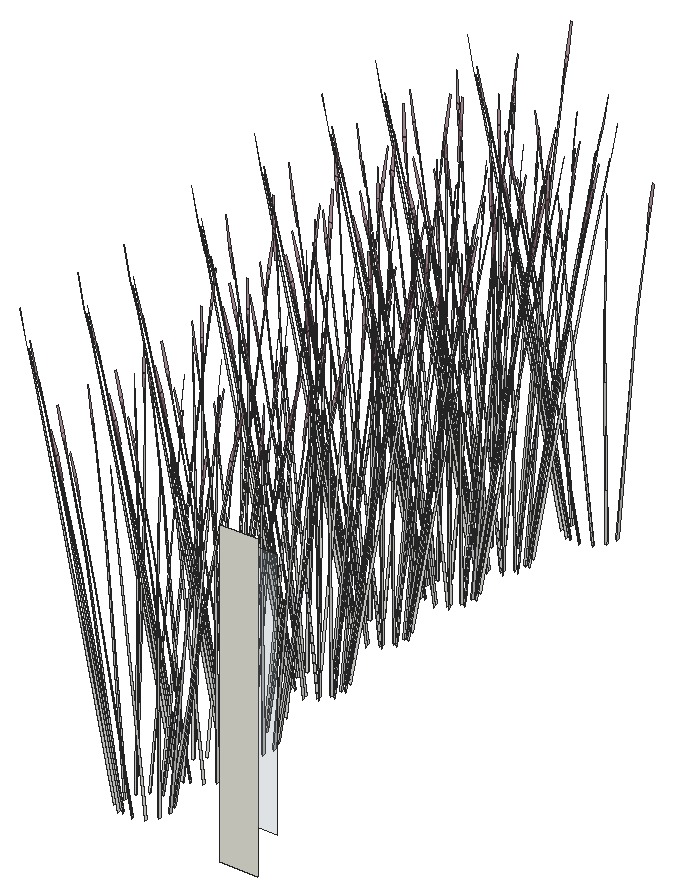
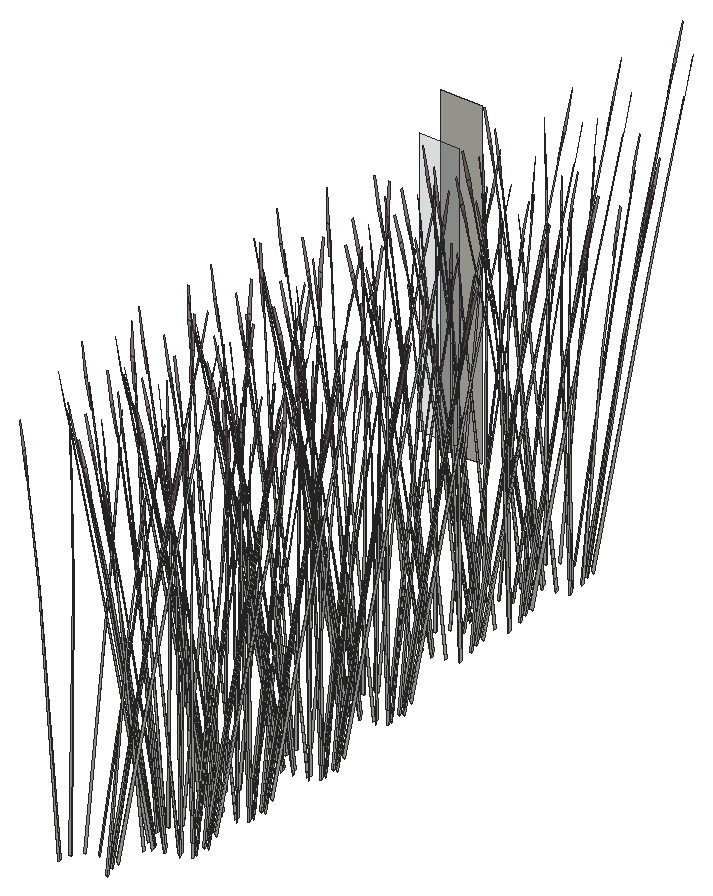
# SketchUp Ruby script. Lengths in inches.
U = 1.inch
M = Sketchup.active_model
def pt(a) = Geom::Point3d.new(a.map { |v| v * U })
def face(e, loops, mat)
  f = e.add_face(loops[0].map { |a| pt(a) })
  loops[1..].each { |l| e.add_face(l.map { |a| pt(a) }).erase! }
  f.material = f.back_material = mat if mat
  f
end
# faces: each face lists its corners as indices into pts; further lists are holes
def faces(e, pts, list, mat = nil) = list.each { |f| face(e, (f[0].is_a?(Array) ? f : [f]).map { |l| l.map { |i| pts[i] } }, mat) }
# xy, xz, yz: faces in a plane at the given z, y or x. An outline is a flat list of corners, or four numbers for a rectangle; further outlines are holes
def ring(l) = l.size == 4 ? [[l[0], l[1]], [l[2], l[1]], [l[2], l[3]], [l[0], l[3]]] : l.each_slice(2).to_a
def flat(e, list, mat, &to3) = list.each { |f| face(e, (f[0].is_a?(Array) ? f : [f]).map { |l| ring(l).map { |u, v| to3.(u, v) } }, mat) }
def xy(e, z, list, mat = nil) = flat(e, list, mat) { |x, y| [x, y, z] }
def xz(e, y, list, mat = nil) = flat(e, list, mat) { |x, z| [x, y, z] }
def yz(e, x, list, mat = nil) = flat(e, list, mat) { |y, z| [x, y, z] }
def lines(e, pts, list) = list.each { |a, b| e.add_line(pt(pts[a]), pt(pts[b])) }
# prism: a flat outline (further loops are holes) pulled along v
def prism(e, loops, v, mat = nil)
  f = face(e, loops, mat); d = Geom::Vector3d.new(v.map { |x| x * U })
  f.pushpull(f.normal.samedirection?(d) ? d.length : -d.length)
end
def box(e, o, s, mat = nil) = prism(e, [[o, [o[0] + s[0], o[1], o[2]], [o[0] + s[0], o[1] + s[1], o[2]], [o[0], o[1] + s[1], o[2]]]], [0, 0, s[2]], mat)
def at(x, y, z, deg = 0) = Geom::Transformation.translation(pt([x, y, z])) * Geom::Transformation.rotation(ORIGIN, Z_AXIS, deg.degrees)
def axes(o, x, y, z) = Geom::Transformation.new([*x, 0, *y, 0, *z, 0, *pt(o).to_a, 1])
def part(name) = M.definitions.add(name)
# library, detail: a bought-in or finely detailed component or shape, given as its bounding box
def library(name, o, s) = part(name).tap { |d| box(d.entities, o, s) }
def detail(e, o, s) = box(e.add_group.entities, o, s)
def put(e, d, t, mat = nil) = e.add_instance(d, t).tap { |i| i.material = mat if mat }
def group(e, t, mat = nil) = e.add_group.tap { |g| g.transformation = t; g.material = mat if mat }.entities
root = M.entities
M.materials.add("D01_Frost_White").color = [238, 238, 227]
M.materials.add("Glass_Basic_01").color = [161, 173, 186]
M.materials["Glass_Basic_01"].alpha = 0.25
M.materials.add("LightPink_Translucent").color = [144, 107, 117]
M.materials["LightPink_Translucent"].alpha = 0.75
c1 = part("blade")
p = [[2.15,0.21,22],[0,0.17,0],[0.09,0.45,0],[2.18,0.31,22],[2.29,0.31,22],[0.38,0.45,0],
  [2.48,0.24,33],[2.49,0.24,33],[2.48,0.22,33]]
faces(c1.entities,p,[[0,1,2,3],[4,5,2,3],[6,3,4,7],[8,0,3,6]])
c2 = part("seeds")
p = [[0.3,-0.1,1.38],[-0.01,-0.03,1.59],[-0.01,-0.03,0.03],[0.14,-0.07,-0.07],[0.29,-0.03,3],[0.15,0.01,3.11]]
faces(c2.entities,p,[[0,1,2,3],[1,0,4,5]],"LightPink_Translucent")
c3 = part("blade with seeds")
put(c3.entities,c1,at(0,0,0))
put(c3.entities,c2,axes([2.4,0.25,30.99],[1.5799,-0.05474,1.17369],[-0.12525,1.92788,0.29478],[-0.07173,-0.02425,1.56792]))
xz(root,373,[[439,156,442,180]],"D01_Frost_White")
xz(root,375,[[439,158,442,178]],"Glass_Basic_01")
put(root,c3,axes([428.4,376.04,154.3],[0.45651,-0.12123,0.45419],[0.07923,0.47555,0.3745],[-0.10736,-0.14016,0.93983]))
put(root,c3,axes([429.43,376.43,154.27],[-0.12355,0.36271,0.29918],[-0.36044,-0.10579,-0.38624],[-0.03305,-0.14603,0.73904]))
put(root,c3,axes([430.21,376.84,154.27],[-0.27728,0.24833,0.29918],[-0.26248,-0.28355,-0.38624],[0.03994,-0.14407,0.73904]))
put(root,c3,axes([428.56,376.49,154.27],[0.06329,0.37991,0.29918],[-0.36182,0.10032,-0.38624],[-0.09718,-0.10887,0.73904]))
put(root,c3,axes([427.48,376.74,154.3],[0.33843,-0.34808,0.45419],[0.29188,0.36965,0.3745],[-0.15878,-0.06421,0.93983]))
put(root,c3,axes([430.6875,377.61,154.27],[-0.35672,0.06741,0.29918],[-0.09419,-0.38534,-0.38624],[0.10222,-0.1035,0.73904]))
put(root,c3,axes([427.84,377,154.27],[0.23317,0.29531,0.29918],[-0.26625,0.27955,-0.38624],[-0.13527,-0.04253,0.73904]))
put(root,c3,axes([430.75,378.53,154.27],[-0.34057,-0.13158,0.29918],[0.09933,-0.38387,-0.38624],[0.13712,-0.0352,0.73904]))
put(root,c3,axes([427.46,377.83,154.27],[0.34057,0.13158,0.29918],[-0.09933,0.38387,-0.38624],[-0.13712,0.0352,0.73904]))
put(root,c3,axes([428.4,381.79,154.3],[0.45651,-0.12123,0.45419],[0.07923,0.47555,0.3745],[-0.10736,-0.14016,0.93983]))
put(root,c3,axes([430.36,379.36,154.27],[-0.23317,-0.29531,0.29918],[0.26625,-0.27955,-0.38624],[0.13527,0.04253,0.73904]))
put(root,c3,axes([429.43,382.18,154.27],[-0.12355,0.36271,0.29918],[-0.36044,-0.10579,-0.38624],[-0.03305,-0.14603,0.73904]))
put(root,c3,axes([430.21,382.59,154.27],[-0.27728,0.24833,0.29918],[-0.26248,-0.28355,-0.38624],[0.03994,-0.14407,0.73904]))
put(root,c3,axes([427.52,378.75,154.27],[0.35672,-0.06741,0.29918],[0.09419,0.38534,-0.38624],[-0.10222,0.1035,0.73904]))
put(root,c3,axes([428.56,382.24,154.27],[0.06329,0.37991,0.29918],[-0.36182,0.10032,-0.38624],[-0.09718,-0.10887,0.73904]))
put(root,c3,axes([427.48,382.49,154.3],[0.33843,-0.34808,0.45419],[0.29188,0.36965,0.3745],[-0.15878,-0.06421,0.93983]))
put(root,c3,axes([426.71,379.85,154.77],[0.36162,0.1259,-0.05481],[-0.11124,0.3875,-0.2485],[-0.05915,0.05883,0.81966]))
put(root,c3,axes([429.64,379.87,154.27],[-0.06329,-0.37991,0.29918],[0.36182,-0.10032,-0.38624],[0.09718,0.10887,0.73904]))
put(root,c3,axes([430.6875,383.35,154.27],[-0.35672,0.06741,0.29918],[-0.09419,-0.38534,-0.38624],[0.10222,-0.1035,0.73904]))
put(root,c3,axes([428,379.52,154.27],[0.27728,-0.24833,0.29918],[0.26248,0.28355,-0.38624],[-0.03994,0.14407,0.73904]))
put(root,c3,axes([428.78,379.93,154.27],[0.12355,-0.36271,0.29918],[0.36044,0.10579,-0.38624],[0.03305,0.14603,0.73904]))
put(root,c3,axes([429.26,381.22,154.77],[0.28319,-0.27058,-0.05481],[0.25948,0.29635,-0.2485],[0.01827,0.08397,0.81966]))
put(root,c3,axes([427.84,382.75,154.27],[0.23317,0.29531,0.29918],[-0.26625,0.27955,-0.38624],[-0.13527,-0.04253,0.73904]))
put(root,c3,axes([428.77,380.23,154.28],[-0.4038,-0.12331,0.45013],[0.13808,-0.40538,0.37115],[0.02427,0.15942,0.93144]))
put(root,c3,axes([430.75,384.28,154.27],[-0.34057,-0.13158,0.29918],[0.09933,-0.38387,-0.38624],[0.13712,-0.0352,0.73904]))
put(root,c3,axes([428.4,386.36,154.3],[0.45651,-0.12123,0.45419],[0.07923,0.47555,0.3745],[-0.10736,-0.14016,0.93983]))
put(root,c3,axes([427.46,383.58,154.27],[0.34057,0.13158,0.29918],[-0.09933,0.38387,-0.38624],[-0.13712,0.0352,0.73904]))
put(root,c3,axes([429.43,386.75,154.27],[-0.12355,0.36271,0.29918],[-0.36044,-0.10579,-0.38624],[-0.03305,-0.14603,0.73904]))
put(root,c3,axes([430.21,387.16,154.27],[-0.27728,0.24833,0.29918],[-0.26248,-0.28355,-0.38624],[0.03994,-0.14407,0.73904]))
put(root,c3,axes([430.36,385.1,154.27],[-0.23317,-0.29531,0.29918],[0.26625,-0.27955,-0.38624],[0.13527,0.04253,0.73904]))
put(root,c3,axes([428.56,386.81,154.27],[0.06329,0.37991,0.29918],[-0.36182,0.10032,-0.38624],[-0.09718,-0.10887,0.73904]))
put(root,c3,axes([427.48,387.06,154.3],[0.33843,-0.34808,0.45419],[0.29188,0.36965,0.3745],[-0.15878,-0.06421,0.93983]))
put(root,c3,axes([430.6875,387.93,154.27],[-0.35672,0.06741,0.29918],[-0.09419,-0.38534,-0.38624],[0.10222,-0.1035,0.73904]))
put(root,c3,axes([427.52,384.5,154.27],[0.35672,-0.06741,0.29918],[0.09419,0.38534,-0.38624],[-0.10222,0.1035,0.73904]))
put(root,c3,axes([426.71,385.6,154.77],[0.36162,0.1259,-0.05481],[-0.11124,0.3875,-0.2485],[-0.05915,0.05883,0.81966]))
put(root,c3,axes([429.64,385.62,154.27],[-0.06329,-0.37991,0.29918],[0.36182,-0.10032,-0.38624],[0.09718,0.10887,0.73904]))
put(root,c3,axes([427.84,387.32,154.27],[0.23317,0.29531,0.29918],[-0.26625,0.27955,-0.38624],[-0.13527,-0.04253,0.73904]))
put(root,c3,axes([428,385.27,154.27],[0.27728,-0.24833,0.29918],[0.26248,0.28355,-0.38624],[-0.03994,0.14407,0.73904]))
put(root,c3,axes([428.78,385.68,154.27],[0.12355,-0.36271,0.29918],[0.36044,0.10579,-0.38624],[0.03305,0.14603,0.73904]))
put(root,c3,axes([430.75,388.85,154.27],[-0.34057,-0.13158,0.29918],[0.09933,-0.38387,-0.38624],[0.13712,-0.0352,0.73904]))
put(root,c3,axes([429.26,386.97,154.77],[0.28319,-0.27058,-0.05481],[0.25948,0.29635,-0.2485],[0.01827,0.08397,0.81966]))
put(root,c3,axes([428.77,385.98,154.28],[-0.4038,-0.12331,0.45013],[0.13808,-0.40538,0.37115],[0.02427,0.15942,0.93144]))
put(root,c3,axes([427.46,388.15,154.27],[0.34057,0.13158,0.29918],[-0.09933,0.38387,-0.38624],[-0.13712,0.0352,0.73904]))
put(root,c3,axes([430.36,389.68,154.27],[-0.23317,-0.29531,0.29918],[0.26625,-0.27955,-0.38624],[0.13527,0.04253,0.73904]))
put(root,c3,axes([427.52,389.07,154.27],[0.35672,-0.06741,0.29918],[0.09419,0.38534,-0.38624],[-0.10222,0.1035,0.73904]))
put(root,c3,axes([426.71,390.17,154.77],[0.36162,0.1259,-0.05481],[-0.11124,0.3875,-0.2485],[-0.05915,0.05883,0.81966]))
put(root,c3,axes([429.64,390.1875,154.27],[-0.06329,-0.37991,0.29918],[0.36182,-0.10032,-0.38624],[0.09718,0.10887,0.73904]))
put(root,c3,axes([428,389.84,154.27],[0.27728,-0.24833,0.29918],[0.26248,0.28355,-0.38624],[-0.03994,0.14407,0.73904]))
put(root,c3,axes([427.05,394.79,154.3],[0.45651,-0.12123,0.45419],[0.07923,0.47555,0.3745],[-0.10736,-0.14016,0.93983]))
put(root,c3,axes([428.08,394.875,154],[0.4038,0.12331,0.40553],[-0.13808,0.40538,0.33437],[-0.02427,-0.15942,0.83914]))
put(root,c3,axes([428.78,390.25,154.27],[0.12355,-0.36271,0.29918],[0.36044,0.10579,-0.38624],[0.03305,0.14603,0.73904]))
put(root,c3,axes([429.26,391.54,154.77],[0.28319,-0.27058,-0.05481],[0.25948,0.29635,-0.2485],[0.01827,0.08397,0.81966]))
put(root,c3,axes([428.07,395.17,154.27],[-0.12355,0.36271,0.29918],[-0.36044,-0.10579,-0.38624],[-0.03305,-0.14603,0.73904]))
put(root,c3,axes([429,395.33,154],[0.29182,0.32181,0.40553],[-0.3099,0.27755,0.33437],[0.05383,-0.15098,0.83914]))
put(root,c3,axes([428.77,390.55,154.28],[-0.4038,-0.12331,0.45013],[0.13808,-0.40538,0.37115],[0.02427,0.15942,0.93144]))
put(root,c3,axes([428.85,395.58,154.27],[-0.27728,0.24833,0.29918],[-0.26248,-0.28355,-0.38624],[0.03994,-0.14407,0.73904]))
put(root,c3,axes([427.21,395.24,154.27],[0.06329,0.37991,0.29918],[-0.36182,0.10032,-0.38624],[-0.09718,-0.10887,0.73904]))
put(root,c3,axes([426.12,395.48,154.3],[0.33843,-0.34808,0.45419],[0.29188,0.36965,0.3745],[-0.15878,-0.06421,0.93983]))
put(root,c3,axes([429.33,396.35,154.27],[-0.35672,0.06741,0.29918],[-0.09419,-0.38534,-0.38624],[0.10222,-0.1035,0.73904]))
put(root,c3,axes([429.58,396.21,154],[0.10163,0.43409,0.40553],[-0.39868,0.07534,0.33437],[0.1175,-0.10209,0.83914]))
put(root,c3,axes([426.49,395.75,154.27],[0.23317,0.29531,0.29918],[-0.26625,0.27955,-0.38624],[-0.13527,-0.04253,0.73904]))
put(root,c3,axes([429.39,397.27,154.27],[-0.34057,-0.13158,0.29918],[0.09933,-0.38387,-0.38624],[0.13712,-0.0352,0.73904]))
put(root,c3,axes([425.82,396.57,154],[0.11578,-0.43006,0.40553],[0.38064,0.14706,0.33437],[-0.14969,0.02584,0.83914]))
put(root,c3,axes([429.67,397.28,154],[-0.11578,0.43006,0.40553],[-0.38064,-0.14706,0.33437],[0.14969,-0.02584,0.83914]))
put(root,c3,axes([426.1,396.58,154.27],[0.34057,0.13158,0.29918],[-0.09933,0.38387,-0.38624],[-0.13712,0.0352,0.73904]))
put(root,c3,axes([429.01,398.1,154.27],[-0.23317,-0.29531,0.29918],[0.26625,-0.27955,-0.38624],[0.13527,0.04253,0.73904]))
put(root,c3,axes([425.92,397.64,154],[-0.10163,-0.43409,0.40553],[0.39868,-0.07534,0.33437],[-0.1175,0.10209,0.83914]))
put(root,c3,axes([426.16,397.5,154.27],[0.35672,-0.06741,0.29918],[0.09419,0.38534,-0.38624],[-0.10222,0.1035,0.73904]))
put(root,c3,axes([429.25,398.25,154],[-0.30217,0.31079,0.40553],[-0.2606,-0.33005,0.33437],[0.14177,0.05733,0.83914]))
put(root,c3,axes([425.96,402.37,154.3],[0.45651,-0.12123,0.45419],[0.07923,0.47555,0.3745],[-0.10736,-0.14016,0.93983]))
put(root,c3,axes([426.99,402.46,154],[0.4038,0.12331,0.40553],[-0.13808,0.40538,0.33437],[-0.02427,-0.15942,0.83914]))
put(root,c3,axes([425.35,398.59,154.77],[0.36162,0.1259,-0.05481],[-0.11124,0.3875,-0.2485],[-0.05915,0.05883,0.81966]))
put(root,c3,axes([428.28,398.61,154.27],[-0.06329,-0.37991,0.29918],[0.36182,-0.10032,-0.38624],[0.09718,0.10887,0.73904]))
put(root,c3,axes([426.64,398.27,154.27],[0.27728,-0.24833,0.29918],[0.26248,0.28355,-0.38624],[-0.03994,0.14407,0.73904]))
put(root,c3,axes([426.99,402.75,154.27],[-0.12355,0.36271,0.29918],[-0.36044,-0.10579,-0.38624],[-0.03305,-0.14603,0.73904]))
put(root,c3,axes([427.91,402.91,154],[0.29182,0.32181,0.40553],[-0.3099,0.27755,0.33437],[0.05383,-0.15098,0.83914]))
put(root,c3,axes([426.5,398.52,154],[-0.29182,-0.32181,0.40553],[0.3099,-0.27755,0.33437],[-0.05383,0.15098,0.83914]))
put(root,c3,axes([427.42,398.67,154.27],[0.12355,-0.36271,0.29918],[0.36044,0.10579,-0.38624],[0.03305,0.14603,0.73904]))
put(root,c3,axes([427.77,403.16,154.27],[-0.27728,0.24833,0.29918],[-0.26248,-0.28355,-0.38624],[0.03994,-0.14407,0.73904]))
put(root,c3,axes([427.9,399.97,154.77],[0.28319,-0.27058,-0.05481],[0.25948,0.29635,-0.2485],[0.01827,0.08397,0.81966]))
put(root,c3,axes([428.42,398.875,154],[-0.4076,0.10824,0.40553],[-0.07074,-0.4246,0.33437],[0.09586,0.12514,0.83914]))
put(root,c3,axes([426.125,402.8125,154.27],[0.06329,0.37991,0.29918],[-0.36182,0.10032,-0.38624],[-0.09718,-0.10887,0.73904]))
put(root,c3,axes([425.04,403.0625,154.3],[0.33843,-0.34808,0.45419],[0.29188,0.36965,0.3745],[-0.15878,-0.06421,0.93983]))
put(root,c3,axes([427.41,398.97,154.28],[-0.4038,-0.12331,0.45013],[0.13808,-0.40538,0.37115],[0.02427,0.15942,0.93144]))
put(root,c3,axes([428.25,403.93,154.27],[-0.35672,0.06741,0.29918],[-0.09419,-0.38534,-0.38624],[0.10222,-0.1035,0.73904]))
put(root,c3,axes([428.49,403.78,154],[0.10163,0.43409,0.40553],[-0.39868,0.07534,0.33437],[0.1175,-0.10209,0.83914]))
put(root,c3,axes([425.4,403.33,154.27],[0.23317,0.29531,0.29918],[-0.26625,0.27955,-0.38624],[-0.13527,-0.04253,0.73904]))
put(root,c3,axes([428.3,404.85,154.27],[-0.34057,-0.13158,0.29918],[0.09933,-0.38387,-0.38624],[0.13712,-0.0352,0.73904]))
put(root,c3,axes([424.74,404.15,154],[0.11578,-0.43006,0.40553],[0.38064,0.14706,0.33437],[-0.14969,0.02584,0.83914]))
put(root,c3,axes([428.58,404.86,154],[-0.11578,0.43006,0.40553],[-0.38064,-0.14706,0.33437],[0.14969,-0.02584,0.83914]))
put(root,c3,axes([425.02,404.15,154.27],[0.34057,0.13158,0.29918],[-0.09933,0.38387,-0.38624],[-0.13712,0.0352,0.73904]))
put(root,c3,axes([427.92,405.68,154.27],[-0.23317,-0.29531,0.29918],[0.26625,-0.27955,-0.38624],[0.13527,0.04253,0.73904]))
put(root,c3,axes([426.11,408.92,154.3],[0.45651,-0.12123,0.45419],[0.07923,0.47555,0.3745],[-0.10736,-0.14016,0.93983]))
put(root,c3,axes([427.14,409,154],[0.4038,0.12331,0.40553],[-0.13808,0.40538,0.33437],[-0.02427,-0.15942,0.83914]))
put(root,c3,axes([424.83,405.22,154],[-0.10163,-0.43409,0.40553],[0.39868,-0.07534,0.33437],[-0.1175,0.10209,0.83914]))
put(root,c3,axes([425.08,405.08,154.27],[0.35672,-0.06741,0.29918],[0.09419,0.38534,-0.38624],[-0.10222,0.1035,0.73904]))
put(root,c3,axes([427.13,409.3,154.27],[-0.12355,0.36271,0.29918],[-0.36044,-0.10579,-0.38624],[-0.03305,-0.14603,0.73904]))
put(root,c3,axes([428.05,409.45,154],[0.29182,0.32181,0.40553],[-0.3099,0.27755,0.33437],[0.05383,-0.15098,0.83914]))
put(root,c3,axes([428.16,405.83,154],[-0.30217,0.31079,0.40553],[-0.2606,-0.33005,0.33437],[0.14177,0.05733,0.83914]))
put(root,c3,axes([427.91,409.71,154.27],[-0.27728,0.24833,0.29918],[-0.26248,-0.28355,-0.38624],[0.03994,-0.14407,0.73904]))
put(root,c3,axes([424.27,406.17,154.77],[0.36162,0.1259,-0.05481],[-0.11124,0.3875,-0.2485],[-0.05915,0.05883,0.81966]))
put(root,c3,axes([427.2,406.19,154.27],[-0.06329,-0.37991,0.29918],[0.36182,-0.10032,-0.38624],[0.09718,0.10887,0.73904]))
put(root,c3,axes([426.27,409.36,154.27],[0.06329,0.37991,0.29918],[-0.36182,0.10032,-0.38624],[-0.09718,-0.10887,0.73904]))
put(root,c3,axes([425.18,409.61,154.3],[0.33843,-0.34808,0.45419],[0.29188,0.36965,0.3745],[-0.15878,-0.06421,0.93983]))
put(root,c3,axes([425.56,405.84,154.27],[0.27728,-0.24833,0.29918],[0.26248,0.28355,-0.38624],[-0.03994,0.14407,0.73904]))
put(root,c3,axes([425.41,406.1,154],[-0.29182,-0.32181,0.40553],[0.3099,-0.27755,0.33437],[-0.05383,0.15098,0.83914]))
put(root,c3,axes([426.34,406.25,154.27],[0.12355,-0.36271,0.29918],[0.36044,0.10579,-0.38624],[0.03305,0.14603,0.73904]))
put(root,c3,axes([428.39,410.48,154.27],[-0.35672,0.06741,0.29918],[-0.09419,-0.38534,-0.38624],[0.10222,-0.1035,0.73904]))
put(root,c3,axes([426.82,407.55,154.77],[0.28319,-0.27058,-0.05481],[0.25948,0.29635,-0.2485],[0.01827,0.08397,0.81966]))
put(root,c3,axes([427.34,406.45,154],[-0.4076,0.10824,0.40553],[-0.07074,-0.4246,0.33437],[0.09586,0.12514,0.83914]))
put(root,c3,axes([428.64,410.33,154],[0.10163,0.43409,0.40553],[-0.39868,0.07534,0.33437],[0.1175,-0.10209,0.83914]))
put(root,c3,axes([426.33,406.55,154.28],[-0.4038,-0.12331,0.45013],[0.13808,-0.40538,0.37115],[0.02427,0.15942,0.93144]))
put(root,c3,axes([425.55,409.875,154.27],[0.23317,0.29531,0.29918],[-0.26625,0.27955,-0.38624],[-0.13527,-0.04253,0.73904]))
put(root,c3,axes([428.45,411.4,154.27],[-0.34057,-0.13158,0.29918],[0.09933,-0.38387,-0.38624],[0.13712,-0.0352,0.73904]))
put(root,c3,axes([424.88,410.7,154],[0.11578,-0.43006,0.40553],[0.38064,0.14706,0.33437],[-0.14969,0.02584,0.83914]))
put(root,c3,axes([428.73,411.4,154],[-0.11578,0.43006,0.40553],[-0.38064,-0.14706,0.33437],[0.14969,-0.02584,0.83914]))
put(root,c3,axes([425.16,410.7,154.27],[0.34057,0.13158,0.29918],[-0.09933,0.38387,-0.38624],[-0.13712,0.0352,0.73904]))
put(root,c3,axes([426.04,414.3,154.3],[0.45651,-0.12123,0.45419],[0.07923,0.47555,0.3745],[-0.10736,-0.14016,0.93983]))
put(root,c3,axes([427.07,414.39,154],[0.4038,0.12331,0.40553],[-0.13808,0.40538,0.33437],[-0.02427,-0.15942,0.83914]))
put(root,c3,axes([428.07,412.23,154.27],[-0.23317,-0.29531,0.29918],[0.26625,-0.27955,-0.38624],[0.13527,0.04253,0.73904]))
put(root,c3,axes([427.0625,414.68,154.27],[-0.12355,0.36271,0.29918],[-0.36044,-0.10579,-0.38624],[-0.03305,-0.14603,0.73904]))
put(root,c3,axes([427.98,414.84,154],[0.29182,0.32181,0.40553],[-0.3099,0.27755,0.33437],[0.05383,-0.15098,0.83914]))
put(root,c3,axes([427.84,415.09,154.27],[-0.27728,0.24833,0.29918],[-0.26248,-0.28355,-0.38624],[0.03994,-0.14407,0.73904]))
put(root,c3,axes([424.98,411.77,154],[-0.10163,-0.43409,0.40553],[0.39868,-0.07534,0.33437],[-0.1175,0.10209,0.83914]))
put(root,c3,axes([426.2,414.74,154.27],[0.06329,0.37991,0.29918],[-0.36182,0.10032,-0.38624],[-0.09718,-0.10887,0.73904]))
put(root,c3,axes([425.11,414.99,154.3],[0.33843,-0.34808,0.45419],[0.29188,0.36965,0.3745],[-0.15878,-0.06421,0.93983]))
put(root,c3,axes([425.22,411.625,154.27],[0.35672,-0.06741,0.29918],[0.09419,0.38534,-0.38624],[-0.10222,0.1035,0.73904]))
put(root,c3,axes([428.31,412.38,154],[-0.30217,0.31079,0.40553],[-0.2606,-0.33005,0.33437],[0.14177,0.05733,0.83914]))
put(root,c3,axes([428.32,415.86,154.27],[-0.35672,0.06741,0.29918],[-0.09419,-0.38534,-0.38624],[0.10222,-0.1035,0.73904]))
put(root,c3,axes([424.41,412.72,154.77],[0.36162,0.1259,-0.05481],[-0.11124,0.3875,-0.2485],[-0.05915,0.05883,0.81966]))
put(root,c3,axes([427.34,412.74,154.27],[-0.06329,-0.37991,0.29918],[0.36182,-0.10032,-0.38624],[0.09718,0.10887,0.73904]))
put(root,c3,axes([428.57,415.72,154],[0.10163,0.43409,0.40553],[-0.39868,0.07534,0.33437],[0.1175,-0.10209,0.83914]))
put(root,c3,axes([425.7,412.39,154.27],[0.27728,-0.24833,0.29918],[0.26248,0.28355,-0.38624],[-0.03994,0.14407,0.73904]))
put(root,c3,axes([425.56,412.65,154],[-0.29182,-0.32181,0.40553],[0.3099,-0.27755,0.33437],[-0.05383,0.15098,0.83914]))
put(root,c3,axes([426.48,412.8,154.27],[0.12355,-0.36271,0.29918],[0.36044,0.10579,-0.38624],[0.03305,0.14603,0.73904]))
put(root,c3,axes([425.48,415.26,154.27],[0.23317,0.29531,0.29918],[-0.26625,0.27955,-0.38624],[-0.13527,-0.04253,0.73904]))
put(root,c3,axes([426.96,414.09,154.77],[0.28319,-0.27058,-0.05481],[0.25948,0.29635,-0.2485],[0.01827,0.08397,0.81966]))
put(root,c3,axes([427.48,413,154],[-0.4076,0.10824,0.40553],[-0.07074,-0.4246,0.33437],[0.09586,0.12514,0.83914]))
put(root,c3,axes([426.47,413.1,154.28],[-0.4038,-0.12331,0.45013],[0.13808,-0.40538,0.37115],[0.02427,0.15942,0.93144]))
put(root,c3,axes([428.38,416.78,154.27],[-0.34057,-0.13158,0.29918],[0.09933,-0.38387,-0.38624],[0.13712,-0.0352,0.73904]))
put(root,c3,axes([424.8125,416.08,154],[0.11578,-0.43006,0.40553],[0.38064,0.14706,0.33437],[-0.14969,0.02584,0.83914]))
put(root,c3,axes([428.66,416.79,154],[-0.11578,0.43006,0.40553],[-0.38064,-0.14706,0.33437],[0.14969,-0.02584,0.83914]))
put(root,c3,axes([425.09,416.09,154.27],[0.34057,0.13158,0.29918],[-0.09933,0.38387,-0.38624],[-0.13712,0.0352,0.73904]))
put(root,c3,axes([428.4,420.45,154.3],[0.45651,-0.12123,0.45419],[0.07923,0.47555,0.3745],[-0.10736,-0.14016,0.93983]))
put(root,c3,axes([428,417.61,154.27],[-0.23317,-0.29531,0.29918],[0.26625,-0.27955,-0.38624],[0.13527,0.04253,0.73904]))
put(root,c3,axes([424.91,417.15,154],[-0.10163,-0.43409,0.40553],[0.39868,-0.07534,0.33437],[-0.1175,0.10209,0.83914]))
put(root,c3,axes([429.43,420.84,154.27],[-0.12355,0.36271,0.29918],[-0.36044,-0.10579,-0.38624],[-0.03305,-0.14603,0.73904]))
put(root,c3,axes([425.15,417.01,154.27],[0.35672,-0.06741,0.29918],[0.09419,0.38534,-0.38624],[-0.10222,0.1035,0.73904]))
put(root,c3,axes([430.21,421.25,154.27],[-0.27728,0.24833,0.29918],[-0.26248,-0.28355,-0.38624],[0.03994,-0.14407,0.73904]))
put(root,c3,axes([428.24,417.76,154],[-0.30217,0.31079,0.40553],[-0.2606,-0.33005,0.33437],[0.14177,0.05733,0.83914]))
put(root,c3,axes([424.34,418.1,154.77],[0.36162,0.1259,-0.05481],[-0.11124,0.3875,-0.2485],[-0.05915,0.05883,0.81966]))
put(root,c3,axes([428.56,420.9,154.27],[0.06329,0.37991,0.29918],[-0.36182,0.10032,-0.38624],[-0.09718,-0.10887,0.73904]))
put(root,c3,axes([427.27,418.12,154.27],[-0.06329,-0.37991,0.29918],[0.36182,-0.10032,-0.38624],[0.09718,0.10887,0.73904]))
put(root,c3,axes([427.48,421.15,154.3],[0.33843,-0.34808,0.45419],[0.29188,0.36965,0.3745],[-0.15878,-0.06421,0.93983]))
put(root,c3,axes([425.63,417.77,154.27],[0.27728,-0.24833,0.29918],[0.26248,0.28355,-0.38624],[-0.03994,0.14407,0.73904]))
put(root,c3,axes([430.6875,422.02,154.27],[-0.35672,0.06741,0.29918],[-0.09419,-0.38534,-0.38624],[0.10222,-0.1035,0.73904]))
put(root,c3,axes([425.49,418.03,154],[-0.29182,-0.32181,0.40553],[0.3099,-0.27755,0.33437],[-0.05383,0.15098,0.83914]))
put(root,c3,axes([426.41,418.18,154.27],[0.12355,-0.36271,0.29918],[0.36044,0.10579,-0.38624],[0.03305,0.14603,0.73904]))
put(root,c3,axes([426.89,419.48,154.77],[0.28319,-0.27058,-0.05481],[0.25948,0.29635,-0.2485],[0.01827,0.08397,0.81966]))
put(root,c3,axes([427.41,418.38,154],[-0.4076,0.10824,0.40553],[-0.07074,-0.4246,0.33437],[0.09586,0.12514,0.83914]))
put(root,c3,axes([426.4,418.48,154.28],[-0.4038,-0.12331,0.45013],[0.13808,-0.40538,0.37115],[0.02427,0.15942,0.93144]))
put(root,c3,axes([427.84,421.41,154.27],[0.23317,0.29531,0.29918],[-0.26625,0.27955,-0.38624],[-0.13527,-0.04253,0.73904]))
put(root,c3,axes([430.75,422.9375,154.27],[-0.34057,-0.13158,0.29918],[0.09933,-0.38387,-0.38624],[0.13712,-0.0352,0.73904]))
put(root,c3,axes([427.46,422.24,154.27],[0.34057,0.13158,0.29918],[-0.09933,0.38387,-0.38624],[-0.13712,0.0352,0.73904]))
